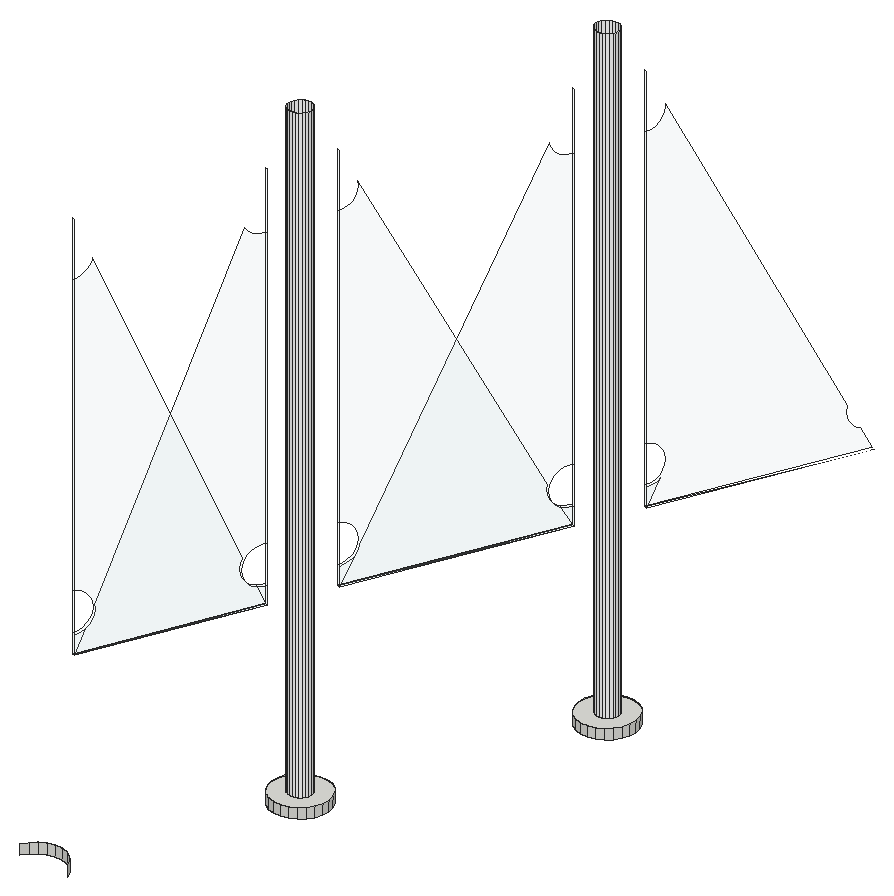
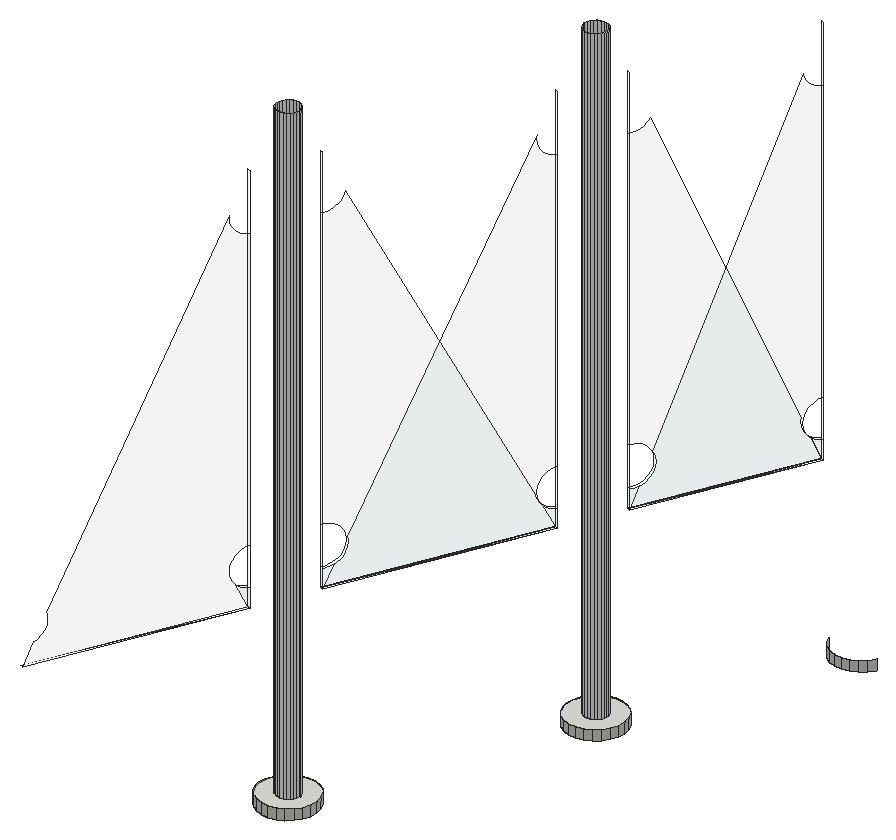
# SketchUp Ruby script. Lengths in inches.
U = 1.inch
M = Sketchup.active_model
def pt(a) = Geom::Point3d.new(a.map { |v| v * U })
def face(e, loops, mat)
  f = e.add_face(loops[0].map { |a| pt(a) })
  loops[1..].each { |l| e.add_face(l.map { |a| pt(a) }).erase! }
  f.material = f.back_material = mat if mat
  f
end
# faces: each face lists its corners as indices into pts; further lists are holes
def faces(e, pts, list, mat = nil) = list.each { |f| face(e, (f[0].is_a?(Array) ? f : [f]).map { |l| l.map { |i| pts[i] } }, mat) }
# xy, xz, yz: faces in a plane at the given z, y or x. An outline is a flat list of corners, or four numbers for a rectangle; further outlines are holes
def ring(l) = l.size == 4 ? [[l[0], l[1]], [l[2], l[1]], [l[2], l[3]], [l[0], l[3]]] : l.each_slice(2).to_a
def flat(e, list, mat, &to3) = list.each { |f| face(e, (f[0].is_a?(Array) ? f : [f]).map { |l| ring(l).map { |u, v| to3.(u, v) } }, mat) }
def xy(e, z, list, mat = nil) = flat(e, list, mat) { |x, y| [x, y, z] }
def xz(e, y, list, mat = nil) = flat(e, list, mat) { |x, z| [x, y, z] }
def yz(e, x, list, mat = nil) = flat(e, list, mat) { |y, z| [x, y, z] }
def lines(e, pts, list) = list.each { |a, b| e.add_line(pt(pts[a]), pt(pts[b])) }
# prism: a flat outline (further loops are holes) pulled along v
def prism(e, loops, v, mat = nil)
  f = face(e, loops, mat); d = Geom::Vector3d.new(v.map { |x| x * U })
  f.pushpull(f.normal.samedirection?(d) ? d.length : -d.length)
end
def box(e, o, s, mat = nil) = prism(e, [[o, [o[0] + s[0], o[1], o[2]], [o[0] + s[0], o[1] + s[1], o[2]], [o[0], o[1] + s[1], o[2]]]], [0, 0, s[2]], mat)
def at(x, y, z, deg = 0) = Geom::Transformation.translation(pt([x, y, z])) * Geom::Transformation.rotation(ORIGIN, Z_AXIS, deg.degrees)
def axes(o, x, y, z) = Geom::Transformation.new([*x, 0, *y, 0, *z, 0, *pt(o).to_a, 1])
def part(name) = M.definitions.add(name)
# library, detail: a bought-in or finely detailed component or shape, given as its bounding box
def library(name, o, s) = part(name).tap { |d| box(d.entities, o, s) }
def detail(e, o, s) = box(e.add_group.entities, o, s)
def put(e, d, t, mat = nil) = e.add_instance(d, t).tap { |i| i.material = mat if mat }
def group(e, t, mat = nil) = e.add_group.tap { |g| g.transformation = t; g.material = mat if mat }.entities
root = M.entities
M.materials.add("Glass_Safety_01").color = [204, 235, 244]
M.materials["Glass_Safety_01"].alpha = 0.1
M.materials.add("[Color_000]").color = [255, 255, 255]
xy(root,321.27,[[[858.75,569.72,859.15,569.81,859.52,569.99,859.83,570.26,860.05,570.61,860.18,571,860.21,571.41,860.125,571.81,859.9375,572.18,859.67,572.48,859.32,572.71,858.93,572.84,858.52,572.86,858.12,572.78,857.75,572.6,857.44,572.33,857.22,571.98,857.09,571.59,857.06,571.18,857.15,570.78,857.33,570.41,857.6,570.1,857.95,569.88,858.34,569.75],[858.68,570.67,858.52,570.68,858.38,570.72,858.36,570.73,858.22,570.82,858.11,570.94,858.04,571.09,858.01,571.25,858.02,571.41,858.07,571.57,858.16,571.71,858.28,571.82,858.43,571.89,858.59,571.92,858.75,571.91,858.89,571.87,858.91,571.86,859.05,571.77,859.16,571.65,859.23,571.5,859.26,571.34,859.25,571.17,859.2,571.02,859.11,570.88,858.99,570.77,858.84,570.7]],[858.01,569.86,858.38,570.72,858.36,570.73,858.22,570.82,858.11,570.94,858.04,571.09,858.01,571.25,858.02,571.41,858.07,571.57,858.16,571.71,858.28,571.82,858.43,571.89,858.59,571.92,858.75,571.91,858.89,571.87,859.26,572.73,858.93,572.84,858.52,572.86,858.12,572.78,857.75,572.6,857.44,572.33,857.22,571.98,857.09,571.59,857.06,571.18,857.15,570.78,857.33,570.41,857.6,570.1,857.95,569.88],[858.38,570.72,858.89,571.87,858.75,571.91,858.59,571.92,858.43,571.89,858.28,571.82,858.16,571.71,858.07,571.57,858.02,571.41,858.01,571.25,858.04,571.09,858.11,570.94,858.22,570.82,858.36,570.73],[[865,584.08,865.4,584.17,865.77,584.35,866.08,584.62,866.31,584.97,866.4375,585.36,866.46,585.77,866.38,586.17,866.19,586.54,865.92,586.84,865.58,587.07,865.52,587.09,865.1875,587.2,864.78,587.22,864.375,587.14,864.01,586.96,863.7,586.69,863.47,586.34,863.34,585.95,863.32,585.54,863.4,585.14,863.59,584.77,863.86,584.46,864.2,584.24,864.59,584.11],[864.93,585.03,864.77,585.04,864.64,585.08,864.61,585.09,864.48,585.18,864.37,585.3,864.29,585.45,864.26,585.61,864.27,585.77,864.32,585.93,864.41,586.07,864.54,586.18,864.68,586.25,864.84,586.28,865.01,586.27,865.14,586.23,865.16,586.22,865.3,586.13,865.41,586.01,865.48,585.86,865.52,585.7,865.51,585.53,865.46,585.38,865.37,585.24,865.24,585.13,865.1,585.06]],[864.26,584.22,864.64,585.08,864.61,585.09,864.48,585.18,864.37,585.3,864.29,585.45,864.26,585.61,864.27,585.77,864.32,585.93,864.41,586.07,864.54,586.18,864.68,586.25,864.84,586.28,865.01,586.27,865.14,586.23,865.52,587.09,865.1875,587.2,864.78,587.22,864.375,587.14,864.01,586.96,863.7,586.69,863.47,586.34,863.34,585.95,863.32,585.54,863.4,585.14,863.59,584.77,863.86,584.46,864.2,584.24],
  [864.64,585.08,865.14,586.23,865.01,586.27,864.84,586.28,864.68,586.25,864.54,586.18,864.41,586.07,864.32,585.93,864.27,585.77,864.26,585.61,864.29,585.45,864.37,585.3,864.48,585.18,864.61,585.09]])
xy(root,321.27,[[858.68,570.67,858.84,570.7,858.99,570.77,859.11,570.88,859.2,571.02,859.25,571.17,859.26,571.34,859.23,571.5,859.16,571.65,859.05,571.77,858.91,571.86,858.89,571.87,858.38,570.72,858.52,570.68],[864.93,585.03,865.1,585.06,865.24,585.13,865.37,585.24,865.46,585.38,865.51,585.53,865.52,585.7,865.48,585.86,865.41,586.01,865.3,586.13,865.16,586.22,865.14,586.23,864.64,585.08,864.77,585.04]],"[Color_000]")
xy(root,321.86,[[858.75,569.72,859.15,569.81,859.52,569.99,859.83,570.26,860.05,570.61,860.18,571,860.21,571.41,860.125,571.81,859.9375,572.18,859.67,572.48,859.32,572.71,858.93,572.84,858.52,572.86,858.12,572.78,857.75,572.6,857.44,572.33,857.22,571.98,857.09,571.59,857.06,571.18,857.15,570.78,857.33,570.41,857.6,570.1,857.95,569.88,858.34,569.75],[865,584.08,865.4,584.17,865.77,584.35,866.08,584.62,866.31,584.97,866.4375,585.36,866.46,585.77,866.38,586.17,866.19,586.54,865.92,586.84,865.58,587.07,865.1875,587.2,864.78,587.22,864.375,587.14,864.01,586.96,863.7,586.69,863.47,586.34,863.34,585.95,863.32,585.54,863.4,585.14,863.59,584.77,863.86,584.46,864.2,584.24,864.59,584.11]])
xy(root,331.9,[[854.11,560.66,853.93,560.73,858.05,569.71],[853.93,560.73,857.875,569.79,858.05,569.71],[859.51,573.06,859.33,573.14,864.29,584.04],[859.33,573.14,864.11,584.12,864.29,584.04],[865.77,587.42,865.59,587.5,870.4,598.07]],"Glass_Safety_01")
p = [[854.72,559.41,321.27],[854.54,559.77,321.27],[854.54,559.77,321.86],[854.72,559.41,321.86],[852.04,559.92,321.27],[851.82,559.58,321.27],
  [851.82,559.58,321.86],[852.04,559.92,321.86],[854.26,560.08,321.27],[854.26,560.08,321.86],[852.35,560.19,321.27],[852.35,560.19,321.86],
  [853.92,560.31,321.27],[853.92,560.31,321.86],[852.72,560.38,321.27],[852.72,560.38,321.86],[853.86,560.33,321.27],[853.53,560.4375,321.27],
  [853.53,560.4375,321.86],[853.12,560.46,321.27],[853.12,560.46,321.86],[857.95,569.88,321.27],[858.01,569.86,321.27],[858.34,569.75,321.27],
  [858.34,569.75,321.86],[857.95,569.88,321.86],[858.75,569.72,321.27],[858.75,569.72,321.86],[859.15,569.81,321.27],[859.15,569.81,321.86],
  [859.52,569.99,321.27],[859.52,569.99,321.86],[857.6,570.1,321.27],[857.6,570.1,321.86],[859.83,570.26,321.27],[859.83,570.26,321.86],
  [857.33,570.41,321.27],[857.33,570.41,321.86],[860.05,570.61,321.27],[860.05,570.61,321.86],[857.15,570.78,321.27],[857.15,570.78,321.86],
  [860.18,571,321.27],[860.18,571,321.86],[858.22,570.82,321.27],[858.36,570.73,321.27],[858.36,570.73,357.27],[858.22,570.82,357.27],
  [858.38,570.72,321.27],[858.52,570.68,321.27],[858.52,570.68,357.27],[858.68,570.67,321.27],[858.68,570.67,357.27],[858.84,570.7,321.27],
  [858.84,570.7,357.27],[858.99,570.77,321.27],[858.99,570.77,357.27],[857.06,571.18,321.27],[857.06,571.18,321.86],[858.11,570.94,321.27],
  [858.11,570.94,357.27],[859.11,570.88,321.27],[859.11,570.88,357.27],[858.04,571.09,321.27],[858.04,571.09,357.27],[859.2,571.02,321.27],
  [859.2,571.02,357.27],[859.25,571.17,321.27],[859.25,571.17,357.27],[860.21,571.41,321.27],[860.21,571.41,321.86],[858.01,571.25,321.27],
  [858.01,571.25,357.27],[857.09,571.59,321.27],[857.09,571.59,321.86],[858.02,571.41,321.27],[858.02,571.41,357.27],[859.26,571.34,321.27],
  [859.26,571.34,357.27],[859.23,571.5,321.27],[859.23,571.5,357.27],[858.07,571.57,321.27],[858.07,571.57,357.27],[860.125,571.81,321.27],
  [860.125,571.81,321.86],[859.16,571.65,321.27],[859.16,571.65,357.27],[857.22,571.98,321.27],[857.22,571.98,321.86],[858.16,571.71,321.27],
  [858.16,571.71,357.27],[859.05,571.77,321.27],[859.05,571.77,357.27],[858.28,571.82,321.27],[858.28,571.82,357.27],[858.43,571.89,321.27],
  [858.43,571.89,357.27],[858.91,571.86,321.27],[858.91,571.86,357.27],[859.9375,572.18,321.27],[859.9375,572.18,321.86],[858.59,571.92,321.27],
  [858.59,571.92,357.27],[858.75,571.91,321.27],[858.75,571.91,357.27],[858.89,571.87,321.27],[857.44,572.33,321.27],[857.44,572.33,321.86],
  [859.67,572.48,321.27],[859.67,572.48,321.86],[857.75,572.6,321.27],[857.75,572.6,321.86],[859.32,572.71,321.27],[859.32,572.71,321.86],
  [858.12,572.78,321.27],[858.12,572.78,321.86],[859.26,572.73,321.27],[858.93,572.84,321.27],[858.93,572.84,321.86],[858.52,572.86,321.27],
  [858.52,572.86,321.86],[864.2,584.24,321.27],[864.26,584.22,321.27],[864.59,584.11,321.27],[864.59,584.11,321.86],[864.2,584.24,321.86],
  [865,584.08,321.27],[865,584.08,321.86],[865.4,584.17,321.27],[865.4,584.17,321.86],[863.86,584.46,321.27],[863.86,584.46,321.86],
  [865.77,584.35,321.27],[865.77,584.35,321.86],[866.08,584.62,321.27],[866.08,584.62,321.86],[863.59,584.77,321.27],[863.59,584.77,321.86],
  [866.31,584.97,321.27],[866.31,584.97,321.86],[863.4,585.14,321.27],[863.4,585.14,321.86],[864.61,585.09,321.27],[864.64,585.08,321.27],
  [864.77,585.04,321.27],[864.77,585.04,357.27],[864.61,585.09,357.27],[864.93,585.03,321.27],[864.93,585.03,357.27],[865.1,585.06,321.27],
  [865.1,585.06,357.27],[866.4375,585.36,321.27],[866.4375,585.36,321.86],[863.32,585.54,321.27],[863.32,585.54,321.86],[864.48,585.18,321.27],
  [864.48,585.18,357.27],[865.24,585.13,321.27],[865.24,585.13,357.27],[865.37,585.24,321.27],[865.37,585.24,357.27],[864.37,585.3,321.27],
  [864.37,585.3,357.27],[865.46,585.38,321.27],[865.46,585.38,357.27],[864.29,585.45,321.27],[864.29,585.45,357.27],[864.26,585.61,321.27],
  [864.26,585.61,357.27],[865.51,585.53,321.27],[865.51,585.53,357.27],[866.46,585.77,321.27],[866.46,585.77,321.86],[863.34,585.95,321.27],
  [863.34,585.95,321.86],[865.52,585.7,321.27],[865.52,585.7,357.27],[864.27,585.77,321.27],[864.27,585.77,357.27],[865.48,585.86,321.27],
  [865.48,585.86,357.27],[864.32,585.93,321.27],[864.32,585.93,357.27],[866.38,586.17,321.27],[866.38,586.17,321.86],[864.41,586.07,321.27],
  [864.41,586.07,357.27],[865.41,586.01,321.27],[865.41,586.01,357.27],[863.47,586.34,321.27],[863.47,586.34,321.86],[865.3,586.13,321.27],
  [865.3,586.13,357.27],[864.54,586.18,321.27],[864.54,586.18,357.27],[865.16,586.22,321.27],[865.16,586.22,357.27],[864.68,586.25,321.27],
  [864.68,586.25,357.27],[864.84,586.28,321.27],[864.84,586.28,357.27],[865.14,586.23,321.27],[865.01,586.27,321.27],[865.01,586.27,357.27],
  [866.19,586.54,321.27],[866.19,586.54,321.86],[863.7,586.69,321.27],[863.7,586.69,321.86],[865.92,586.84,321.27],[865.92,586.84,321.86],
  [864.01,586.96,321.27],[864.01,586.96,321.86],[865.58,587.07,321.27],[865.58,587.07,321.86],[864.375,587.14,321.27],[864.375,587.14,321.86],
  [864.78,587.22,321.27],[864.78,587.22,321.86],[865.52,587.09,321.27],[865.1875,587.2,321.27],[865.1875,587.2,321.86],[853.93,560.73,331.9],
  [854.11,560.66,331.9],[854.11,560.66,333],[854.11,560.66,335.125],[854.11,560.66,351.28],[854.11,560.66,353.41],[854.11,560.66,354.51],
  [853.93,560.73,354.51],[853.93,560.73,353.41],[853.93,560.73,351.28],[853.93,560.73,335.125],[853.93,560.73,333],[854.04,560.99,333.04],
  [854.14,561.22,333.14],[854.23,561.42,333.3125],[854.3,561.58,333.53],[854.34,561.68,333.79],[854.35,561.71,334.0625],[854.34,561.68,334.34],
  [854.3,561.58,334.59],[854.23,561.42,334.8125],[854.14,561.22,334.98],[854.04,560.99,335.09],[854.04,560.99,351.32],[854.14,561.22,351.43],
  [854.23,561.42,351.59],[854.3,561.58,351.81],[854.34,561.68,352.07],[854.34,561.68,352.14],[857.4,568.7,334.62],[857.39,568.68,334.59],
  [857.35,568.59,334.34],[857.33,568.55,334.0625],[857.35,568.59,333.79],[857.39,568.68,333.53],[857.46,568.84,333.3125],[857.55,569.04,333.14],
  [857.65,569.28,333.04],[857.68,569.34,333.03],[857.875,569.79,331.9],[854.33,561.16,333.16],[854.32,561.14,333.14],[854.22,560.91,333.04],
  [858.05,569.71,335.125],[858.05,569.71,351.28],[857.9375,569.45,351.28],[857.83,569.2,351.32],[857.73,568.96,351.43],[857.64,568.76,351.59],
  [857.58,568.62,351.79],[854.52,561.61,334.27],[854.53,561.63,334.0625],[854.52,561.6,333.79],[854.48,561.5,333.53],[854.41,561.35,333.3125],
  [858.05,569.71,331.9],[858.05,569.71,333],[857.9375,569.45,333],[857.83,569.2,333.04],[857.73,568.96,333.14],[857.64,568.76,333.3125],
  [857.57,568.61,333.53],[857.53,568.51,333.79],[857.52,568.48,334.0625],[857.53,568.51,334.34],[857.57,568.61,334.59],[857.64,568.76,334.8125],
  [857.73,568.96,334.98],[857.83,569.2,335.09],[857.9375,569.45,335.125],[857.76,569.53,333],[857.875,569.79,333],[857.875,569.79,335.125],
  [857.875,569.79,351.28],[857.875,569.79,353.41],[857.875,569.79,354.51],[858.05,569.71,354.51],[858.05,569.71,353.41],[859.33,573.14,331.9],
  [859.51,573.06,331.9],[859.51,573.06,333],[859.51,573.06,335.125],[859.51,573.06,351.28],[859.51,573.06,353.41],[859.51,573.06,354.51],
  [859.33,573.14,354.51],[859.33,573.14,353.41],[859.33,573.14,351.28],[859.33,573.14,335.125],[859.33,573.14,333],[859.74,574.09,352.56],
  [863.6,582.94,334.3125],[863.59,582.91,334.0625],[863.6,582.95,333.79],[863.65,583.04,333.53],[863.71,583.2,333.3125],[863.8,583.4,333.14],
  [863.86,583.54,333.08],[864.11,584.12,331.9],[859.44,573.39,333.04],[859.54,573.625,333.14],[859.63,573.83,333.3125],[859.7,573.98,333.53],
  [859.74,574.08,333.79],[859.76,574.11,334.0625],[859.74,574.08,334.34],[859.7,573.98,334.59],[859.63,573.83,334.8125],[859.54,573.625,334.98],
  [859.44,573.39,335.09],[859.44,573.39,351.32],[859.54,573.625,351.43],[859.63,573.83,351.59],[859.7,573.98,351.81],[859.74,574.08,352.07],
  [859.76,574.11,352.35],[859.81,573.74,333.31],[859.72,573.55,333.14],[859.62,573.3125,333.04],[864.29,584.04,335.125],[864.29,584.04,351.28],
  [864.19,583.81,351.28],[864.08,583.56,351.32],[863.98,583.32,351.43],[863.89,583.12,351.59],[863.83,582.97,351.81],[863.78,582.87,352.07],
  [863.78,582.87,352.1],[859.92,574.01,333.85],[859.92,574,333.79],[859.88,573.9,333.53],[859.8125,573.75,333.3125],[864.29,584.04,331.9],
  [864.29,584.04,333],[864.19,583.81,333],[864.08,583.56,333.04],[863.98,583.32,333.14],[863.89,583.12,333.3125],[863.83,582.97,333.53],
  [863.78,582.87,333.79],[863.77,582.84,334.0625],[863.78,582.87,334.34],[863.83,582.97,334.59],[863.89,583.12,334.8125],[863.98,583.32,334.98],
  [864.08,583.56,335.09],[864.19,583.81,335.125],[863.9,583.64,333.04],[864.01,583.89,333],[864.11,584.12,333],[864.11,584.12,335.125],
  [864.11,584.12,351.28],[864.11,584.12,353.41],[864.11,584.12,354.51],[864.29,584.04,354.51],[864.29,584.04,353.41],[865.59,587.5,331.9],
  [865.77,587.42,331.9],[865.77,587.42,333],[865.77,587.42,335.125],[865.77,587.42,351.28],[865.77,587.42,353.41],[865.77,587.42,354.51],
  [865.59,587.5,354.51],[865.59,587.5,353.41],[865.59,587.5,351.28],[865.59,587.5,335.125],[865.59,587.5,333],[866.05,588.07,333.28],
  [865.98,587.91,333.14],[865.875,587.67,333.04],[866,588.46,352.47],[869.72,596.99,334.37],[869.71,596.97,334.34],[869.7,596.94,334.0625],
  [869.71,596.97,333.79],[869.75,597.07,333.53],[869.82,597.23,333.3125],[869.91,597.43,333.14],[869.98,597.6,333.07],[870.22,598.15,331.9],
  [865.7,587.75,333.04],[865.8,587.99,333.14],[865.89,588.1875,333.3125],[865.95,588.34,333.53],[866,588.4375,333.79],[866.01,588.47,334.0625],
  [866,588.4375,334.34],[865.95,588.34,334.59],[865.89,588.1875,334.8125],[865.8,587.99,334.98],[865.7,587.75,335.09],[865.7,587.75,351.32],
  [865.8,587.99,351.43],[865.89,588.1875,351.59],[865.95,588.34,351.81],[866,588.4375,352.07],[866.01,588.47,352.35]]
faces(root,p,[[0,1,2,3],[4,5,6,7],[1,8,9,2],[10,4,7,11],[8,12,13,9],[14,10,11,15],[12,16,17,18,13],[19,14,15,20],
  [17,19,20,18],[21,22,23,24,25],[23,26,27,24],[26,28,29,27],[28,30,31,29],[32,21,25,33],[30,34,35,31],[36,32,33,37],
  [34,38,39,35],[40,36,37,41],[38,42,43,39],[57,40,41,58],[42,69,70,43],[73,57,58,74],[69,83,84,70],[87,73,74,88],
  [83,99,100,84],[106,87,88,107],[99,108,109,100],[110,106,107,111],[108,112,113,109],[114,110,111,115],[112,116,117,118,113],[119,114,115,120],
  [117,119,120,118],[121,122,123,124,125],[123,126,127,124],[126,128,129,127],[130,121,125,131],[128,132,133,129],[132,134,135,133],[136,130,131,137],
  [134,138,139,135],[140,136,137,141],[138,151,152,139],[153,140,141,154],[151,171,172,152],[173,153,154,174],[171,183,184,172],[189,173,174,190],
  [183,204,205,184],[206,189,190,207],[204,208,209,205],[210,206,207,211],[208,212,213,209],[214,210,211,215],[216,214,215,217],[212,218,219,220,213],
  [219,216,217,220]])
faces(root,p,[[44,45,46,47],[45,48,49,50,46],[49,51,52,50],[51,53,54,52],[53,55,56,54],[59,44,47,60],[55,61,62,56],[63,59,60,64],
  [61,65,66,62],[65,67,68,66],[71,63,64,72],[75,71,72,76],[67,77,78,68],[77,79,80,78],[81,75,76,82],[79,85,86,80],
  [89,81,82,90],[85,91,92,86],[93,89,90,94],[95,93,94,96],[91,97,98,92],[101,95,96,102],[103,101,102,104],[97,105,103,104,98],
  [142,143,144,145,146],[144,147,148,145],[147,149,150,148],[155,142,146,156],[149,157,158,150],[157,159,160,158],[161,155,156,162],[159,163,164,160],
  [165,161,162,166],[167,165,166,168],[163,169,170,164],[169,175,176,170],[177,167,168,178],[175,179,180,176],[181,177,178,182],[185,181,182,186],
  [179,187,188,180],[187,191,192,188],[193,185,186,194],[191,195,196,192],[197,193,194,198],[199,197,198,200],[195,201,202,203,196],[202,199,200,203]],"[Color_000]")
faces(root,p,[[221,222,223,224,225,226,227,228,229,230,231,232],[221,232,233,234,235,236,237,238,239,240,241,242,243,231,230,244,245,246,247,248,249,250,251,252,253,254,255,256,257,258,259,260],[222,261,262,263,223],[264,265,266,267,268,269,270,271,272,273,274,275,261,222,276,277,278,279,280,281,282,283,284,285,286,287,288,289,290],[260,259,291,292],[276,260,292,293,294,295,296,297,298,265,264,277],[299,300,301,302,303,304,305,306,307,308,309,310],[311,312,313,314,315,316,317,318,319,299,310,320,321,322,323,324,325,326,327,328,329,330,309,308,331,332,333,334,335,336],
  [300,337,338,339,301],[340,341,342,343,344,345,346,347,348,349,350,351,352,337,300,353,354,355,356,357,358,359,360,361,362,363,364,365,366,367],[319,318,368,369,370],[353,319,370,371,372,373,374,375,376,341,340,354],[377,378,379,380,381,382,383,384,385,386,387,388],[378,389,390,391,379],[392,393,394,395,396,397,398,399,400,401,377,388,402,403,404,405,406,407,408,409,410,411,412,387,386,413,414,415,416,417,418]],"Glass_Safety_01")
